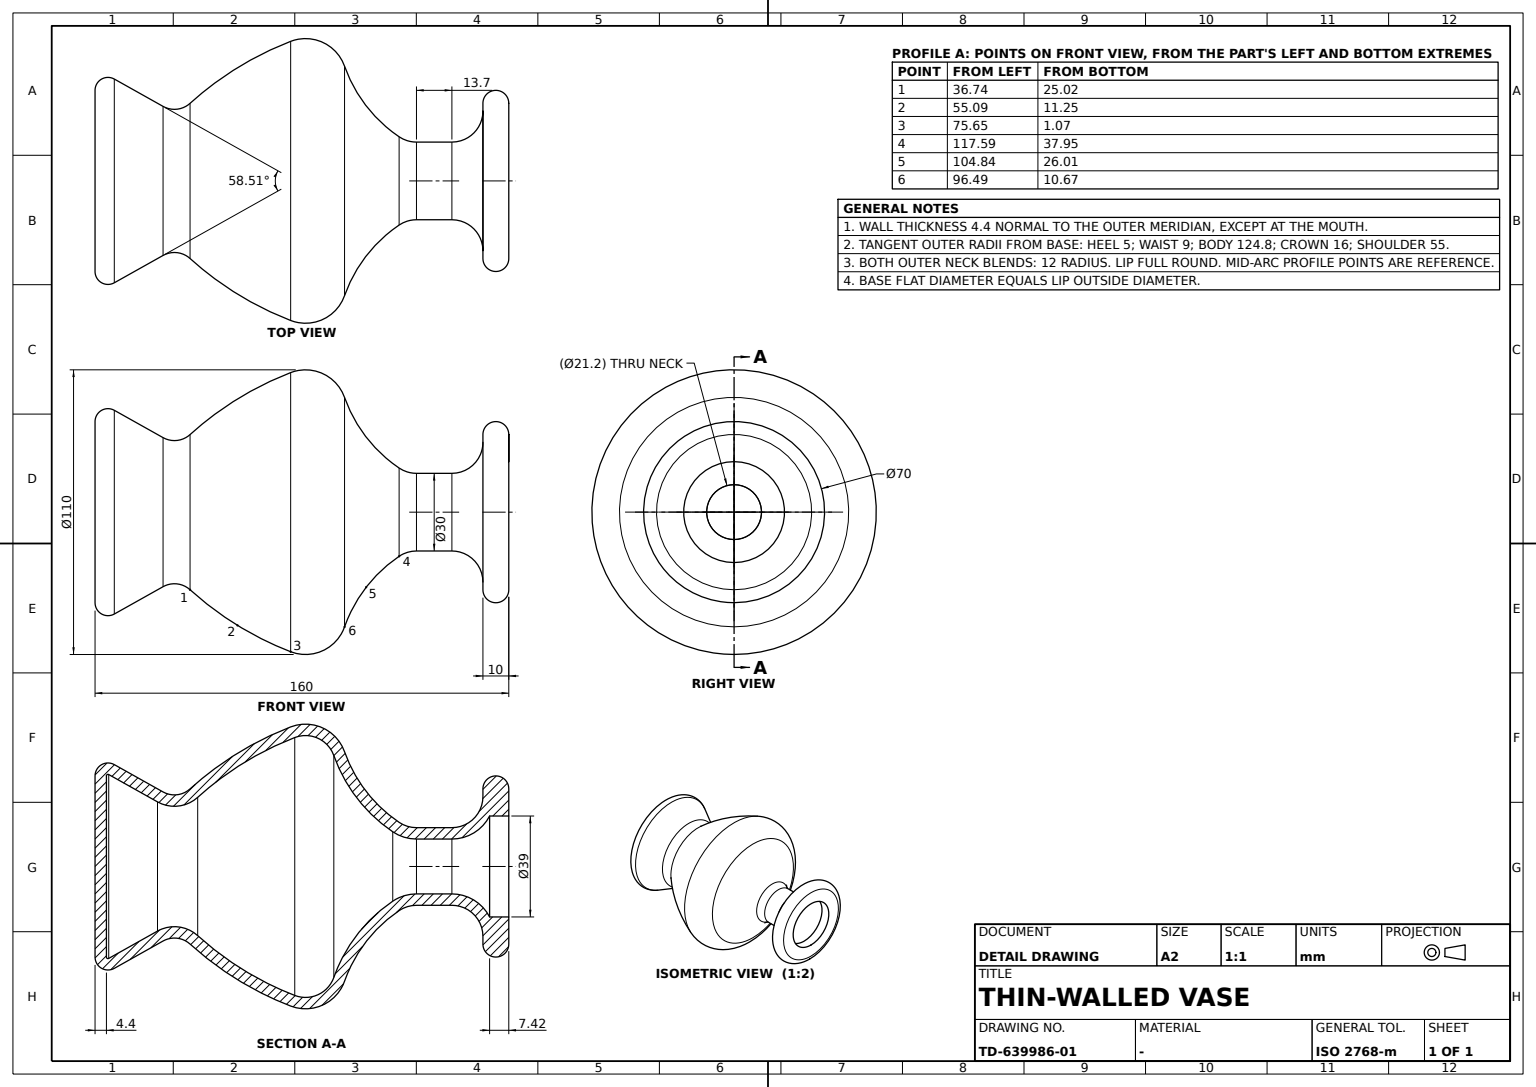
ISO-10303-21;
HEADER;
FILE_DESCRIPTION((''),'2;1');
FILE_NAME('','',(''),(''),'','','');
FILE_SCHEMA(('AUTOMOTIVE_DESIGN'));
ENDSEC;
DATA;
#1=APPLICATION_CONTEXT('');
#2=PRODUCT_CONTEXT('',#1,'mechanical');
#3=PRODUCT('','','',(#2));
#4=PRODUCT_DEFINITION_FORMATION('','',#3);
#5=PRODUCT_DEFINITION_CONTEXT('',#1,'design');
#6=PRODUCT_DEFINITION('','',#4,#5);
#7=PRODUCT_DEFINITION_SHAPE('','',#6);
#8=(LENGTH_UNIT()NAMED_UNIT(*)SI_UNIT(.MILLI.,.METRE.));
#9=(NAMED_UNIT(*)PLANE_ANGLE_UNIT()SI_UNIT($,.RADIAN.));
#10=(NAMED_UNIT(*)SI_UNIT($,.STERADIAN.)SOLID_ANGLE_UNIT());
#11=UNCERTAINTY_MEASURE_WITH_UNIT(LENGTH_MEASURE(0.005),#8,'distance_accuracy_value','');
#12=(GEOMETRIC_REPRESENTATION_CONTEXT(3)GLOBAL_UNCERTAINTY_ASSIGNED_CONTEXT((#11))GLOBAL_UNIT_ASSIGNED_CONTEXT((#8,#9,#10))REPRESENTATION_CONTEXT('',''));
#13=CARTESIAN_POINT('',(44.32916,0.,96.486419));
#14=VERTEX_POINT('',#13);
#15=CARTESIAN_POINT('',(0.,0.,96.486419));
#16=DIRECTION('',(0.,0.,1.));
#17=DIRECTION('',(1.,0.,0.));
#18=AXIS2_PLACEMENT_3D('',#15,#16,#17);
#19=CIRCLE('',#18,44.32916);
#20=EDGE_CURVE('',#14,#14,#19,.T.);
#21=ORIENTED_EDGE('',*,*,#20,.T.);
#22=EDGE_LOOP('',(#21));
#23=FACE_BOUND('',#22,.T.);
#24=CARTESIAN_POINT('',(17.051679,0.,117.589492));
#25=VERTEX_POINT('',#24);
#26=CARTESIAN_POINT('',(0.,0.,117.589492));
#27=AXIS2_PLACEMENT_3D('',#26,#16,#17);
#28=CIRCLE('',#27,17.051679);
#29=EDGE_CURVE('',#25,#25,#28,.T.);
#30=ORIENTED_EDGE('',*,*,#29,.F.);
#31=EDGE_LOOP('',(#30));
#32=FACE_BOUND('',#31,.T.);
#33=CARTESIAN_POINT('',(0.,0.,148.345986));
#34=AXIS2_PLACEMENT_3D('',#33,#16,#17);
#35=TOROIDAL_SURFACE('',#34,62.64815,55.);
#36=ADVANCED_FACE('',(#23,#32),#35,.F.);
#37=CARTESIAN_POINT('',(29.978967,0.,36.741301));
#38=VERTEX_POINT('',#37);
#39=CARTESIAN_POINT('',(0.,0.,36.741301));
#40=AXIS2_PLACEMENT_3D('',#39,#16,#17);
#41=CIRCLE('',#40,29.978967);
#42=EDGE_CURVE('',#38,#38,#41,.T.);
#43=ORIENTED_EDGE('',*,*,#42,.T.);
#44=EDGE_LOOP('',(#43));
#45=FACE_BOUND('',#44,.T.);
#46=CARTESIAN_POINT('',(53.930299,0.,75.647941));
#47=VERTEX_POINT('',#46);
#48=CARTESIAN_POINT('',(0.,0.,75.647941));
#49=AXIS2_PLACEMENT_3D('',#48,#16,#17);
#50=CIRCLE('',#49,53.930299);
#51=EDGE_CURVE('',#47,#47,#50,.T.);
#52=ORIENTED_EDGE('',*,*,#51,.F.);
#53=EDGE_LOOP('',(#52));
#54=FACE_BOUND('',#53,.T.);
#55=CARTESIAN_POINT('',(-28.418018,11.771128,36.741301));
#56=CARTESIAN_POINT('',(-30.759441,0.,36.741301));
#57=CARTESIAN_POINT('',(-28.418018,-11.771128,36.741301));
#58=CARTESIAN_POINT('',(-21.750209,-21.750209,36.741301));
#59=CARTESIAN_POINT('',(-11.771128,-28.418018,36.741301));
#60=CARTESIAN_POINT('',(0.,-30.759441,36.741301));
#61=CARTESIAN_POINT('',(11.771128,-28.418018,36.741301));
#62=CARTESIAN_POINT('',(21.750209,-21.750209,36.741301));
#63=CARTESIAN_POINT('',(28.418018,-11.771128,36.741301));
#64=CARTESIAN_POINT('',(30.759441,0.,36.741301));
#65=CARTESIAN_POINT('',(28.418018,11.771128,36.741301));
#66=CARTESIAN_POINT('',(21.750209,21.750209,36.741301));
#67=CARTESIAN_POINT('',(11.771128,28.418018,36.741301));
#68=CARTESIAN_POINT('',(0.,30.759441,36.741301));
#69=CARTESIAN_POINT('',(-11.771128,28.418018,36.741301));
#70=CARTESIAN_POINT('',(-21.750209,21.750209,36.741301));
#71=CARTESIAN_POINT('',(-33.29123,13.789679,42.417077));
#72=CARTESIAN_POINT('',(-36.034168,0.,42.417077));
#73=CARTESIAN_POINT('',(-33.29123,-13.789679,42.417077));
#74=CARTESIAN_POINT('',(-25.480005,-25.480005,42.417077));
#75=CARTESIAN_POINT('',(-13.789679,-33.29123,42.417077));
#76=CARTESIAN_POINT('',(0.,-36.034168,42.417077));
#77=CARTESIAN_POINT('',(13.789679,-33.29123,42.417077));
#78=CARTESIAN_POINT('',(25.480005,-25.480005,42.417077));
#79=CARTESIAN_POINT('',(33.29123,-13.789679,42.417077));
#80=CARTESIAN_POINT('',(36.034168,0.,42.417077));
#81=CARTESIAN_POINT('',(33.29123,13.789679,42.417077));
#82=CARTESIAN_POINT('',(25.480005,25.480005,42.417077));
#83=CARTESIAN_POINT('',(13.789679,33.29123,42.417077));
#84=CARTESIAN_POINT('',(0.,36.034168,42.417077));
#85=CARTESIAN_POINT('',(-13.789679,33.29123,42.417077));
#86=CARTESIAN_POINT('',(-25.480005,25.480005,42.417077));
#87=CARTESIAN_POINT('',(-42.042261,17.414475,54.719045));
#88=CARTESIAN_POINT('',(-45.506216,0.,54.719045));
#89=CARTESIAN_POINT('',(-42.042261,-17.414475,54.719045));
#90=CARTESIAN_POINT('',(-32.177754,-32.177754,54.719045));
#91=CARTESIAN_POINT('',(-17.414475,-42.042261,54.719045));
#92=CARTESIAN_POINT('',(0.,-45.506216,54.719045));
#93=CARTESIAN_POINT('',(17.414475,-42.042261,54.719045));
#94=CARTESIAN_POINT('',(32.177754,-32.177754,54.719045));
#95=CARTESIAN_POINT('',(42.042261,-17.414475,54.719045));
#96=CARTESIAN_POINT('',(45.506216,0.,54.719045));
#97=CARTESIAN_POINT('',(42.042261,17.414475,54.719045));
#98=CARTESIAN_POINT('',(32.177754,32.177754,54.719045));
#99=CARTESIAN_POINT('',(17.414475,42.042261,54.719045));
#100=CARTESIAN_POINT('',(0.,45.506216,54.719045));
#101=CARTESIAN_POINT('',(-17.414475,42.042261,54.719045));
#102=CARTESIAN_POINT('',(-32.177754,32.177754,54.719045));
#103=CARTESIAN_POINT('',(-48.513144,20.094802,68.501797));
#104=CARTESIAN_POINT('',(-52.510249,0.,68.501797));
#105=CARTESIAN_POINT('',(-48.513144,-20.094802,68.501797));
#106=CARTESIAN_POINT('',(-37.130353,-37.130353,68.501797));
#107=CARTESIAN_POINT('',(-20.094802,-48.513144,68.501797));
#108=CARTESIAN_POINT('',(0.,-52.510249,68.501797));
#109=CARTESIAN_POINT('',(20.094802,-48.513144,68.501797));
#110=CARTESIAN_POINT('',(37.130353,-37.130353,68.501797));
#111=CARTESIAN_POINT('',(48.513144,-20.094802,68.501797));
#112=CARTESIAN_POINT('',(52.510249,0.,68.501797));
#113=CARTESIAN_POINT('',(48.513144,20.094802,68.501797));
#114=CARTESIAN_POINT('',(37.130353,37.130353,68.501797));
#115=CARTESIAN_POINT('',(20.094802,48.513144,68.501797));
#116=CARTESIAN_POINT('',(0.,52.510249,68.501797));
#117=CARTESIAN_POINT('',(-20.094802,48.513144,68.501797));
#118=CARTESIAN_POINT('',(-37.130353,37.130353,68.501797));
#119=CARTESIAN_POINT('',(-51.122249,21.175529,75.647941));
#120=CARTESIAN_POINT('',(-55.334323,0.,75.647941));
#121=CARTESIAN_POINT('',(-51.122249,-21.175529,75.647941));
#122=CARTESIAN_POINT('',(-39.127275,-39.127275,75.647941));
#123=CARTESIAN_POINT('',(-21.175529,-51.122249,75.647941));
#124=CARTESIAN_POINT('',(0.,-55.334323,75.647941));
#125=CARTESIAN_POINT('',(21.175529,-51.122249,75.647941));
#126=CARTESIAN_POINT('',(39.127275,-39.127275,75.647941));
#127=CARTESIAN_POINT('',(51.122249,-21.175529,75.647941));
#128=CARTESIAN_POINT('',(55.334323,0.,75.647941));
#129=CARTESIAN_POINT('',(51.122249,21.175529,75.647941));
#130=CARTESIAN_POINT('',(39.127275,39.127275,75.647941));
#131=CARTESIAN_POINT('',(21.175529,51.122249,75.647941));
#132=CARTESIAN_POINT('',(0.,55.334323,75.647941));
#133=CARTESIAN_POINT('',(-21.175529,51.122249,75.647941));
#134=CARTESIAN_POINT('',(-39.127275,39.127275,75.647941));
#135=B_SPLINE_SURFACE_WITH_KNOTS('',3,3,((#55,#56,#57,#58,#59,#60,#61,#62,#63,#64,#65,#66,#67,#68,#69,#70,#55,#56,#57),(#71,#72,#73,#74,#75,#76,#77,#78,#79,#80,#81,#82,#83,#84,#85,#86,#71,#72,#73),(#87,#88,#89,#90,#91,#92,#93,#94,#95,#96,#97,#98,#99,#100,#101,#102,#87,#88,#89),(#103,#104,#105,#106,#107,#108,#109,#110,#111,#112,#113,#114,#115,#116,#117,#118,#103,#104,#105),(#119,#120,#121,#122,#123,#124,#125,#126,#127,#128,#129,#130,#131,#132,#133,#134,#119,#120,#121)),.UNSPECIFIED.,.F.,.T.,.F.,(4,1,4),(1,1,1,1,1,1,1,1,1,1,1,1,1,1,1,1,1,1,1,1,1,1,1),(5.547283834,5.731366581,5.915449328),(-1.178097245,-0.785398163,-0.392699082,0.,0.392699082,0.785398163,1.178097245,1.570796327,1.963495408,2.35619449,2.748893572,3.141592654,3.534291735,3.926990817,4.319689899,4.71238898,5.105088062,5.497787144,5.890486225,6.283185307,6.675884389,7.068583471,7.461282552),.UNSPECIFIED.);
#136=ADVANCED_FACE('',(#45,#54),#135,.F.);
#137=ORIENTED_EDGE('',*,*,#29,.T.);
#138=EDGE_LOOP('',(#137));
#139=FACE_BOUND('',#138,.T.);
#140=CARTESIAN_POINT('',(15.,0.,124.3));
#141=VERTEX_POINT('',#140);
#142=CARTESIAN_POINT('',(0.,0.,124.3));
#143=AXIS2_PLACEMENT_3D('',#142,#16,#17);
#144=CIRCLE('',#143,15.);
#145=EDGE_CURVE('',#141,#141,#144,.T.);
#146=ORIENTED_EDGE('',*,*,#145,.F.);
#147=EDGE_LOOP('',(#146));
#148=FACE_BOUND('',#147,.T.);
#149=TOROIDAL_SURFACE('',#143,27.,12.);
#150=ADVANCED_FACE('',(#139,#148),#149,.F.);
#151=CARTESIAN_POINT('',(10.6,0.,138.));
#152=VERTEX_POINT('',#151);
#153=CARTESIAN_POINT('',(0.,0.,138.));
#154=AXIS2_PLACEMENT_3D('',#153,#16,#17);
#155=CIRCLE('',#154,10.6);
#156=EDGE_CURVE('',#152,#152,#155,.T.);
#157=ORIENTED_EDGE('',*,*,#156,.T.);
#158=EDGE_LOOP('',(#157));
#159=FACE_BOUND('',#158,.T.);
#160=CARTESIAN_POINT('',(10.6,0.,124.3));
#161=VERTEX_POINT('',#160);
#162=CIRCLE('',#143,10.6);
#163=EDGE_CURVE('',#161,#161,#162,.T.);
#164=ORIENTED_EDGE('',*,*,#163,.F.);
#165=EDGE_LOOP('',(#164));
#166=FACE_BOUND('',#165,.T.);
#167=CARTESIAN_POINT('',(0.,0.,80.));
#168=AXIS2_PLACEMENT_3D('',#167,#16,#17);
#169=CYLINDRICAL_SURFACE('',#168,10.6);
#170=ADVANCED_FACE('',(#159,#166),#169,.F.);
#171=CARTESIAN_POINT('',(35.,0.,0.));
#172=VERTEX_POINT('',#171);
#173=CARTESIAN_POINT('',(0.,0.,0.));
#174=AXIS2_PLACEMENT_3D('',#173,#16,#17);
#175=CIRCLE('',#174,35.);
#176=EDGE_CURVE('',#172,#172,#175,.T.);
#177=ORIENTED_EDGE('',*,*,#176,.T.);
#178=EDGE_LOOP('',(#177));
#179=FACE_BOUND('',#178,.T.);
#180=CARTESIAN_POINT('',(39.362162,0.,7.443674));
#181=VERTEX_POINT('',#180);
#182=CARTESIAN_POINT('',(0.,0.,7.443674));
#183=AXIS2_PLACEMENT_3D('',#182,#16,#17);
#184=CIRCLE('',#183,39.362162);
#185=EDGE_CURVE('',#181,#181,#184,.T.);
#186=ORIENTED_EDGE('',*,*,#185,.F.);
#187=EDGE_LOOP('',(#186));
#188=FACE_BOUND('',#187,.T.);
#189=CARTESIAN_POINT('',(0.,0.,5.));
#190=AXIS2_PLACEMENT_3D('',#189,#16,#17);
#191=TOROIDAL_SURFACE('',#190,35.,5.);
#192=ADVANCED_FACE('',(#179,#188),#191,.T.);
#193=CARTESIAN_POINT('',(27.,0.,150.));
#194=VERTEX_POINT('',#193);
#195=CARTESIAN_POINT('',(0.,0.,150.));
#196=AXIS2_PLACEMENT_3D('',#195,#16,#17);
#197=CIRCLE('',#196,27.);
#198=EDGE_CURVE('',#194,#194,#197,.T.);
#199=ORIENTED_EDGE('',*,*,#198,.F.);
#200=EDGE_LOOP('',(#199));
#201=FACE_BOUND('',#200,.T.);
#202=CARTESIAN_POINT('',(15.,0.,138.));
#203=VERTEX_POINT('',#202);
#204=CIRCLE('',#154,15.);
#205=EDGE_CURVE('',#203,#203,#204,.T.);
#206=ORIENTED_EDGE('',*,*,#205,.T.);
#207=EDGE_LOOP('',(#206));
#208=FACE_BOUND('',#207,.T.);
#209=TOROIDAL_SURFACE('',#154,27.,12.);
#210=ADVANCED_FACE('',(#201,#208),#209,.F.);
#211=CARTESIAN_POINT('',(35.,0.,4.4));
#212=VERTEX_POINT('',#211);
#213=CARTESIAN_POINT('',(0.,0.,4.4));
#214=AXIS2_PLACEMENT_3D('',#213,#16,#17);
#215=CIRCLE('',#214,35.);
#216=EDGE_CURVE('',#212,#212,#215,.T.);
#217=ORIENTED_EDGE('',*,*,#216,.T.);
#218=EDGE_LOOP('',(#217));
#219=FACE_BOUND('',#218,.T.);
#220=PLANE('',#214);
#221=ADVANCED_FACE('',(#219),#220,.T.);
#222=ORIENTED_EDGE('',*,*,#20,.F.);
#223=EDGE_LOOP('',(#222));
#224=FACE_BOUND('',#223,.T.);
#225=ORIENTED_EDGE('',*,*,#51,.T.);
#226=EDGE_LOOP('',(#225));
#227=FACE_BOUND('',#226,.T.);
#228=CARTESIAN_POINT('',(0.,0.,81.4));
#229=AXIS2_PLACEMENT_3D('',#228,#16,#17);
#230=TOROIDAL_SURFACE('',#229,39.,16.);
#231=ADVANCED_FACE('',(#224,#227),#230,.T.);
#232=ORIENTED_EDGE('',*,*,#185,.T.);
#233=EDGE_LOOP('',(#232));
#234=FACE_BOUND('',#233,.T.);
#235=CARTESIAN_POINT('',(28.798109,0.,26.301386));
#236=VERTEX_POINT('',#235);
#237=CARTESIAN_POINT('',(0.,0.,26.301386));
#238=AXIS2_PLACEMENT_3D('',#237,#16,#17);
#239=CIRCLE('',#238,28.798109);
#240=EDGE_CURVE('',#236,#236,#239,.T.);
#241=ORIENTED_EDGE('',*,*,#240,.F.);
#242=EDGE_LOOP('',(#241));
#243=FACE_BOUND('',#242,.T.);
#244=DIRECTION('',(0.,0.,-1.));
#245=AXIS2_PLACEMENT_3D('',#237,#244,#17);
#246=CONICAL_SURFACE('',#245,28.798108829,0.510639065);
#247=ADVANCED_FACE('',(#234,#243),#246,.T.);
#248=CARTESIAN_POINT('',(30.,0.,150.));
#249=VERTEX_POINT('',#248);
#250=CIRCLE('',#196,30.);
#251=EDGE_CURVE('',#249,#249,#250,.T.);
#252=ORIENTED_EDGE('',*,*,#251,.F.);
#253=EDGE_LOOP('',(#252));
#254=FACE_BOUND('',#253,.T.);
#255=ORIENTED_EDGE('',*,*,#198,.T.);
#256=EDGE_LOOP('',(#255));
#257=FACE_BOUND('',#256,.T.);
#258=CARTESIAN_POINT('',(-30.,0.,150.));
#259=AXIS2_PLACEMENT_3D('',#258,#16,#17);
#260=PLANE('',#259);
#261=ADVANCED_FACE('',(#254,#257),#260,.F.);
#262=ORIENTED_EDGE('',*,*,#240,.T.);
#263=EDGE_LOOP('',(#262));
#264=FACE_BOUND('',#263,.T.);
#265=ORIENTED_EDGE('',*,*,#42,.F.);
#266=EDGE_LOOP('',(#265));
#267=FACE_BOUND('',#266,.T.);
#268=CARTESIAN_POINT('',(0.,0.,30.7));
#269=AXIS2_PLACEMENT_3D('',#268,#16,#17);
#270=TOROIDAL_SURFACE('',#269,36.65,9.);
#271=ADVANCED_FACE('',(#264,#267),#270,.F.);
#272=CARTESIAN_POINT('',(42.863641,0.,92.337654));
#273=VERTEX_POINT('',#272);
#274=CARTESIAN_POINT('',(0.,0.,92.337654));
#275=AXIS2_PLACEMENT_3D('',#274,#16,#17);
#276=CIRCLE('',#275,42.863641);
#277=EDGE_CURVE('',#273,#273,#276,.T.);
#278=ORIENTED_EDGE('',*,*,#277,.F.);
#279=EDGE_LOOP('',(#278));
#280=FACE_BOUND('',#279,.T.);
#281=CARTESIAN_POINT('',(13.403962,0.,115.128973));
#282=VERTEX_POINT('',#281);
#283=CARTESIAN_POINT('',(0.,0.,115.128973));
#284=AXIS2_PLACEMENT_3D('',#283,#16,#17);
#285=CIRCLE('',#284,13.403962);
#286=EDGE_CURVE('',#282,#282,#285,.T.);
#287=ORIENTED_EDGE('',*,*,#286,.T.);
#288=EDGE_LOOP('',(#287));
#289=FACE_BOUND('',#288,.T.);
#290=TOROIDAL_SURFACE('',#34,62.64815,59.4);
#291=ADVANCED_FACE('',(#280,#289),#290,.T.);
#292=CARTESIAN_POINT('',(30.,0.,160.));
#293=VERTEX_POINT('',#292);
#294=CARTESIAN_POINT('',(0.,0.,160.));
#295=AXIS2_PLACEMENT_3D('',#294,#16,#17);
#296=CIRCLE('',#295,30.);
#297=EDGE_CURVE('',#293,#293,#296,.T.);
#298=ORIENTED_EDGE('',*,*,#297,.F.);
#299=EDGE_LOOP('',(#298));
#300=FACE_BOUND('',#299,.T.);
#301=ORIENTED_EDGE('',*,*,#251,.T.);
#302=EDGE_LOOP('',(#301));
#303=FACE_BOUND('',#302,.T.);
#304=CARTESIAN_POINT('',(0.,0.,155.));
#305=AXIS2_PLACEMENT_3D('',#304,#16,#17);
#306=TOROIDAL_SURFACE('',#305,30.,5.);
#307=ADVANCED_FACE('',(#300,#303),#306,.T.);
#308=CARTESIAN_POINT('',(26.717572,0.,39.694825));
#309=VERTEX_POINT('',#308);
#310=CARTESIAN_POINT('',(0.,0.,39.694825));
#311=AXIS2_PLACEMENT_3D('',#310,#16,#17);
#312=CIRCLE('',#311,26.717572);
#313=EDGE_CURVE('',#309,#309,#312,.T.);
#314=ORIENTED_EDGE('',*,*,#313,.F.);
#315=EDGE_LOOP('',(#314));
#316=FACE_BOUND('',#315,.T.);
#317=CARTESIAN_POINT('',(49.824466,0.,77.229757));
#318=VERTEX_POINT('',#317);
#319=CARTESIAN_POINT('',(0.,0.,77.229757));
#320=AXIS2_PLACEMENT_3D('',#319,#16,#17);
#321=CIRCLE('',#320,49.824466);
#322=EDGE_CURVE('',#318,#318,#321,.T.);
#323=ORIENTED_EDGE('',*,*,#322,.T.);
#324=EDGE_LOOP('',(#323));
#325=FACE_BOUND('',#324,.T.);
#326=CARTESIAN_POINT('',(-25.326438,10.490554,39.694825));
#327=CARTESIAN_POINT('',(-27.413139,0.,39.694825));
#328=CARTESIAN_POINT('',(-25.326438,-10.490554,39.694825));
#329=CARTESIAN_POINT('',(-19.384017,-19.384017,39.694825));
#330=CARTESIAN_POINT('',(-10.490554,-25.326438,39.694825));
#331=CARTESIAN_POINT('',(0.,-27.413139,39.694825));
#332=CARTESIAN_POINT('',(10.490554,-25.326438,39.694825));
#333=CARTESIAN_POINT('',(19.384017,-19.384017,39.694825));
#334=CARTESIAN_POINT('',(25.326438,-10.490554,39.694825));
#335=CARTESIAN_POINT('',(27.413139,0.,39.694825));
#336=CARTESIAN_POINT('',(25.326438,10.490554,39.694825));
#337=CARTESIAN_POINT('',(19.384017,19.384017,39.694825));
#338=CARTESIAN_POINT('',(10.490554,25.326438,39.694825));
#339=CARTESIAN_POINT('',(0.,27.413139,39.694825));
#340=CARTESIAN_POINT('',(-10.490554,25.326438,39.694825));
#341=CARTESIAN_POINT('',(-19.384017,19.384017,39.694825));
#342=CARTESIAN_POINT('',(-30.027839,12.437938,45.170494));
#343=CARTESIAN_POINT('',(-32.501899,0.,45.170494));
#344=CARTESIAN_POINT('',(-30.027839,-12.437938,45.170494));
#345=CARTESIAN_POINT('',(-22.982313,-22.982313,45.170494));
#346=CARTESIAN_POINT('',(-12.437938,-30.027839,45.170494));
#347=CARTESIAN_POINT('',(0.,-32.501899,45.170494));
#348=CARTESIAN_POINT('',(12.437938,-30.027839,45.170494));
#349=CARTESIAN_POINT('',(22.982313,-22.982313,45.170494));
#350=CARTESIAN_POINT('',(30.027839,-12.437938,45.170494));
#351=CARTESIAN_POINT('',(32.501899,0.,45.170494));
#352=CARTESIAN_POINT('',(30.027839,12.437938,45.170494));
#353=CARTESIAN_POINT('',(22.982313,22.982313,45.170494));
#354=CARTESIAN_POINT('',(12.437938,30.027839,45.170494));
#355=CARTESIAN_POINT('',(0.,32.501899,45.170494));
#356=CARTESIAN_POINT('',(-12.437938,30.027839,45.170494));
#357=CARTESIAN_POINT('',(-22.982313,22.982313,45.170494));
#358=CARTESIAN_POINT('',(-38.47034,15.934937,57.038739));
#359=CARTESIAN_POINT('',(-41.639996,0.,57.038739));
#360=CARTESIAN_POINT('',(-38.47034,-15.934937,57.038739));
#361=CARTESIAN_POINT('',(-29.443924,-29.443924,57.038739));
#362=CARTESIAN_POINT('',(-15.934937,-38.47034,57.038739));
#363=CARTESIAN_POINT('',(0.,-41.639996,57.038739));
#364=CARTESIAN_POINT('',(15.934937,-38.47034,57.038739));
#365=CARTESIAN_POINT('',(29.443924,-29.443924,57.038739));
#366=CARTESIAN_POINT('',(38.47034,-15.934937,57.038739));
#367=CARTESIAN_POINT('',(41.639996,0.,57.038739));
#368=CARTESIAN_POINT('',(38.47034,15.934937,57.038739));
#369=CARTESIAN_POINT('',(29.443924,29.443924,57.038739));
#370=CARTESIAN_POINT('',(15.934937,38.47034,57.038739));
#371=CARTESIAN_POINT('',(0.,41.639996,57.038739));
#372=CARTESIAN_POINT('',(-15.934937,38.47034,57.038739));
#373=CARTESIAN_POINT('',(-29.443924,29.443924,57.038739));
#374=CARTESIAN_POINT('',(-44.713083,18.520765,70.335561));
#375=CARTESIAN_POINT('',(-48.397092,0.,70.335561));
#376=CARTESIAN_POINT('',(-44.713083,-18.520765,70.335561));
#377=CARTESIAN_POINT('',(-34.221912,-34.221912,70.335561));
#378=CARTESIAN_POINT('',(-18.520765,-44.713083,70.335561));
#379=CARTESIAN_POINT('',(0.,-48.397092,70.335561));
#380=CARTESIAN_POINT('',(18.520765,-44.713083,70.335561));
#381=CARTESIAN_POINT('',(34.221912,-34.221912,70.335561));
#382=CARTESIAN_POINT('',(44.713083,-18.520765,70.335561));
#383=CARTESIAN_POINT('',(48.397092,0.,70.335561));
#384=CARTESIAN_POINT('',(44.713083,18.520765,70.335561));
#385=CARTESIAN_POINT('',(34.221912,34.221912,70.335561));
#386=CARTESIAN_POINT('',(18.520765,44.713083,70.335561));
#387=CARTESIAN_POINT('',(0.,48.397092,70.335561));
#388=CARTESIAN_POINT('',(-18.520765,44.713083,70.335561));
#389=CARTESIAN_POINT('',(-34.221912,34.221912,70.335561));
#390=CARTESIAN_POINT('',(-47.2302,19.563389,77.229757));
#391=CARTESIAN_POINT('',(-51.1216,0.,77.229757));
#392=CARTESIAN_POINT('',(-47.2302,-19.563389,77.229757));
#393=CARTESIAN_POINT('',(-36.14843,-36.14843,77.229757));
#394=CARTESIAN_POINT('',(-19.563389,-47.2302,77.229757));
#395=CARTESIAN_POINT('',(0.,-51.1216,77.229757));
#396=CARTESIAN_POINT('',(19.563389,-47.2302,77.229757));
#397=CARTESIAN_POINT('',(36.14843,-36.14843,77.229757));
#398=CARTESIAN_POINT('',(47.2302,-19.563389,77.229757));
#399=CARTESIAN_POINT('',(51.1216,0.,77.229757));
#400=CARTESIAN_POINT('',(47.2302,19.563389,77.229757));
#401=CARTESIAN_POINT('',(36.14843,36.14843,77.229757));
#402=CARTESIAN_POINT('',(19.563389,47.2302,77.229757));
#403=CARTESIAN_POINT('',(0.,51.1216,77.229757));
#404=CARTESIAN_POINT('',(-19.563389,47.2302,77.229757));
#405=CARTESIAN_POINT('',(-36.14843,36.14843,77.229757));
#406=B_SPLINE_SURFACE_WITH_KNOTS('',3,3,((#326,#327,#328,#329,#330,#331,#332,#333,#334,#335,#336,#337,#338,#339,#340,#341,#326,#327,#328),(#342,#343,#344,#345,#346,#347,#348,#349,#350,#351,#352,#353,#354,#355,#356,#357,#342,#343,#344),(#358,#359,#360,#361,#362,#363,#364,#365,#366,#367,#368,#369,#370,#371,#372,#373,#358,#359,#360),(#374,#375,#376,#377,#378,#379,#380,#381,#382,#383,#384,#385,#386,#387,#388,#389,#374,#375,#376),(#390,#391,#392,#393,#394,#395,#396,#397,#398,#399,#400,#401,#402,#403,#404,#405,#390,#391,#392)),.UNSPECIFIED.,.F.,.T.,.F.,(4,1,4),(1,1,1,1,1,1,1,1,1,1,1,1,1,1,1,1,1,1,1,1,1,1,1),(5.547283834,5.731366581,5.915449328),(-1.178097245,-0.785398163,-0.392699082,0.,0.392699082,0.785398163,1.178097245,1.570796327,1.963495408,2.35619449,2.748893572,3.141592654,3.534291735,3.926990817,4.319689899,4.71238898,5.105088062,5.497787144,5.890486225,6.283185307,6.675884389,7.068583471,7.461282552),.UNSPECIFIED.);
#407=ADVANCED_FACE('',(#316,#325),#406,.T.);
#408=ORIENTED_EDGE('',*,*,#145,.T.);
#409=EDGE_LOOP('',(#408));
#410=FACE_BOUND('',#409,.T.);
#411=ORIENTED_EDGE('',*,*,#205,.F.);
#412=EDGE_LOOP('',(#411));
#413=FACE_BOUND('',#412,.T.);
#414=CYLINDRICAL_SURFACE('',#168,15.);
#415=ADVANCED_FACE('',(#410,#413),#414,.T.);
#416=ORIENTED_EDGE('',*,*,#156,.F.);
#417=EDGE_LOOP('',(#416));
#418=FACE_BOUND('',#417,.T.);
#419=CARTESIAN_POINT('',(19.5,0.,152.584581));
#420=VERTEX_POINT('',#419);
#421=CARTESIAN_POINT('',(0.,0.,152.584581));
#422=AXIS2_PLACEMENT_3D('',#421,#16,#17);
#423=CIRCLE('',#422,19.5);
#424=EDGE_CURVE('',#420,#420,#423,.T.);
#425=ORIENTED_EDGE('',*,*,#424,.T.);
#426=EDGE_LOOP('',(#425));
#427=FACE_BOUND('',#426,.T.);
#428=TOROIDAL_SURFACE('',#154,27.,16.4);
#429=ADVANCED_FACE('',(#418,#427),#428,.T.);
#430=ORIENTED_EDGE('',*,*,#216,.F.);
#431=EDGE_LOOP('',(#430));
#432=FACE_BOUND('',#431,.T.);
#433=CARTESIAN_POINT('',(35.523459,0.,5.293241));
#434=VERTEX_POINT('',#433);
#435=CARTESIAN_POINT('',(0.,0.,5.293241));
#436=AXIS2_PLACEMENT_3D('',#435,#16,#17);
#437=CIRCLE('',#436,35.523459);
#438=EDGE_CURVE('',#434,#434,#437,.T.);
#439=ORIENTED_EDGE('',*,*,#438,.T.);
#440=EDGE_LOOP('',(#439));
#441=FACE_BOUND('',#440,.T.);
#442=TOROIDAL_SURFACE('',#190,35.,0.6);
#443=ADVANCED_FACE('',(#432,#441),#442,.F.);
#444=ORIENTED_EDGE('',*,*,#438,.F.);
#445=EDGE_LOOP('',(#444));
#446=FACE_BOUND('',#445,.T.);
#447=CARTESIAN_POINT('',(24.959406,0.,24.150953));
#448=VERTEX_POINT('',#447);
#449=CARTESIAN_POINT('',(0.,0.,24.150953));
#450=AXIS2_PLACEMENT_3D('',#449,#16,#17);
#451=CIRCLE('',#450,24.959406);
#452=EDGE_CURVE('',#448,#448,#451,.T.);
#453=ORIENTED_EDGE('',*,*,#452,.T.);
#454=EDGE_LOOP('',(#453));
#455=FACE_BOUND('',#454,.T.);
#456=AXIS2_PLACEMENT_3D('',#449,#244,#17);
#457=CONICAL_SURFACE('',#456,24.959406479,0.510639065);
#458=ADVANCED_FACE('',(#446,#455),#457,.F.);
#459=ORIENTED_EDGE('',*,*,#297,.T.);
#460=EDGE_LOOP('',(#459));
#461=FACE_BOUND('',#460,.T.);
#462=CARTESIAN_POINT('',(19.5,0.,160.));
#463=VERTEX_POINT('',#462);
#464=CIRCLE('',#295,19.5);
#465=EDGE_CURVE('',#463,#463,#464,.T.);
#466=ORIENTED_EDGE('',*,*,#465,.F.);
#467=EDGE_LOOP('',(#466));
#468=FACE_BOUND('',#467,.T.);
#469=CARTESIAN_POINT('',(-19.5,0.,160.));
#470=AXIS2_PLACEMENT_3D('',#469,#16,#17);
#471=PLANE('',#470);
#472=ADVANCED_FACE('',(#461,#468),#471,.T.);
#473=ORIENTED_EDGE('',*,*,#452,.F.);
#474=EDGE_LOOP('',(#473));
#475=FACE_BOUND('',#474,.T.);
#476=ORIENTED_EDGE('',*,*,#313,.T.);
#477=EDGE_LOOP('',(#476));
#478=FACE_BOUND('',#477,.T.);
#479=TOROIDAL_SURFACE('',#269,36.65,13.4);
#480=ADVANCED_FACE('',(#475,#478),#479,.T.);
#481=ORIENTED_EDGE('',*,*,#176,.F.);
#482=EDGE_LOOP('',(#481));
#483=FACE_BOUND('',#482,.T.);
#484=PLANE('',#174);
#485=ADVANCED_FACE('',(#483),#484,.F.);
#486=ORIENTED_EDGE('',*,*,#465,.T.);
#487=EDGE_LOOP('',(#486));
#488=FACE_BOUND('',#487,.T.);
#489=ORIENTED_EDGE('',*,*,#424,.F.);
#490=EDGE_LOOP('',(#489));
#491=FACE_BOUND('',#490,.T.);
#492=CYLINDRICAL_SURFACE('',#168,19.5);
#493=ADVANCED_FACE('',(#488,#491),#492,.F.);
#494=ORIENTED_EDGE('',*,*,#163,.T.);
#495=EDGE_LOOP('',(#494));
#496=FACE_BOUND('',#495,.T.);
#497=ORIENTED_EDGE('',*,*,#286,.F.);
#498=EDGE_LOOP('',(#497));
#499=FACE_BOUND('',#498,.T.);
#500=TOROIDAL_SURFACE('',#143,27.,16.4);
#501=ADVANCED_FACE('',(#496,#499),#500,.T.);
#502=ORIENTED_EDGE('',*,*,#322,.F.);
#503=EDGE_LOOP('',(#502));
#504=FACE_BOUND('',#503,.T.);
#505=ORIENTED_EDGE('',*,*,#277,.T.);
#506=EDGE_LOOP('',(#505));
#507=FACE_BOUND('',#506,.T.);
#508=TOROIDAL_SURFACE('',#229,39.,11.6);
#509=ADVANCED_FACE('',(#504,#507),#508,.F.);
#510=CLOSED_SHELL('',(#36,#136,#150,#170,#192,#210,#221,#231,#247,#261,#271,#291,#307,#407,#415,#429,#443,#458,#472,#480,#485,#493,#501,#509));
#511=MANIFOLD_SOLID_BREP('',#510);
#512=ADVANCED_BREP_SHAPE_REPRESENTATION('',(#511),#12);
#513=SHAPE_DEFINITION_REPRESENTATION(#7,#512);
ENDSEC;
END-ISO-10303-21;
